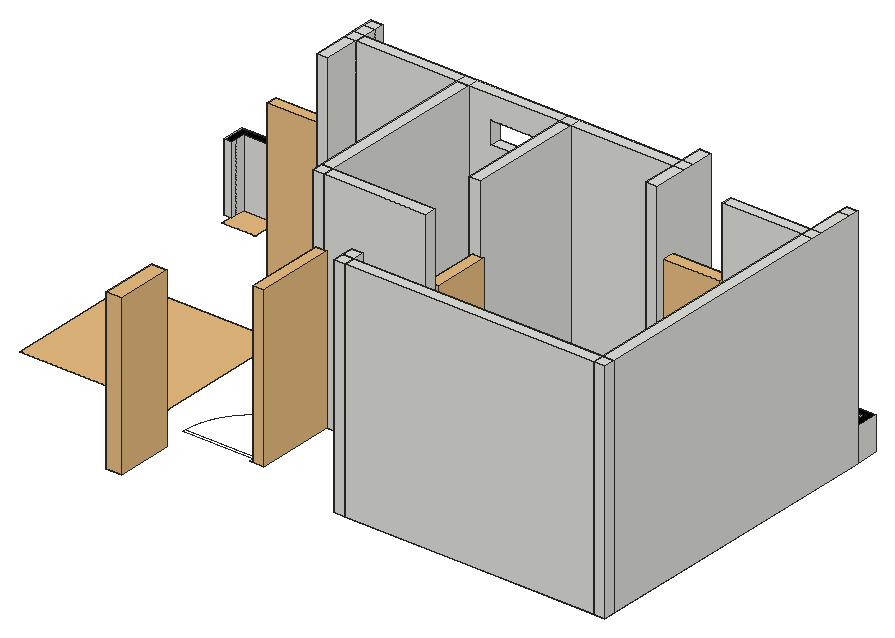
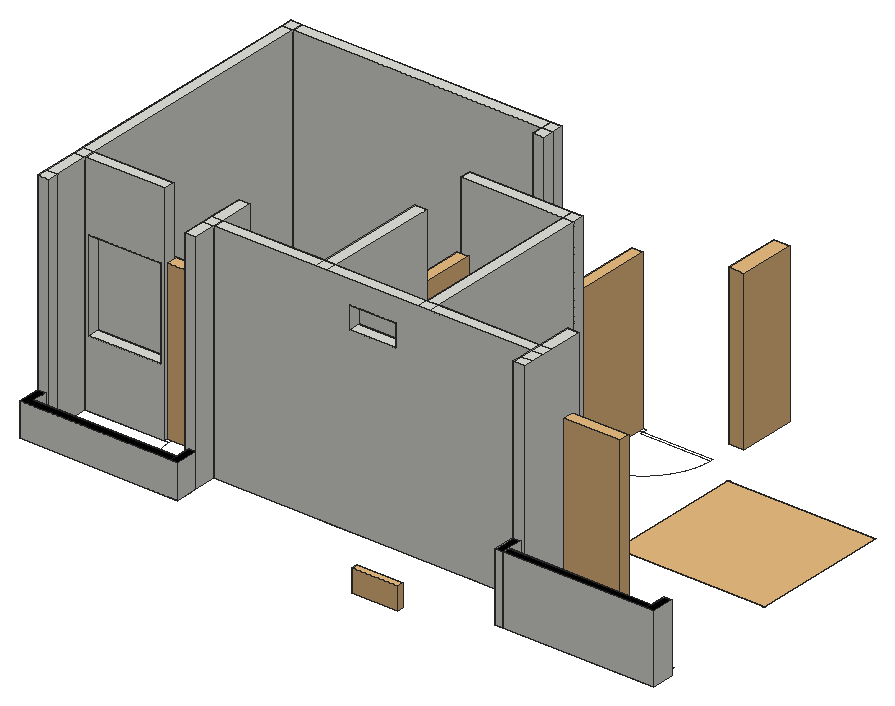
# SketchUp Ruby script. Lengths in inches.
U = 1.inch
M = Sketchup.active_model
def pt(a) = Geom::Point3d.new(a.map { |v| v * U })
def face(e, loops, mat)
  f = e.add_face(loops[0].map { |a| pt(a) })
  loops[1..].each { |l| e.add_face(l.map { |a| pt(a) }).erase! }
  f.material = f.back_material = mat if mat
  f
end
# faces: each face lists its corners as indices into pts; further lists are holes
def faces(e, pts, list, mat = nil) = list.each { |f| face(e, (f[0].is_a?(Array) ? f : [f]).map { |l| l.map { |i| pts[i] } }, mat) }
# xy, xz, yz: faces in a plane at the given z, y or x. An outline is a flat list of corners, or four numbers for a rectangle; further outlines are holes
def ring(l) = l.size == 4 ? [[l[0], l[1]], [l[2], l[1]], [l[2], l[3]], [l[0], l[3]]] : l.each_slice(2).to_a
def flat(e, list, mat, &to3) = list.each { |f| face(e, (f[0].is_a?(Array) ? f : [f]).map { |l| ring(l).map { |u, v| to3.(u, v) } }, mat) }
def xy(e, z, list, mat = nil) = flat(e, list, mat) { |x, y| [x, y, z] }
def xz(e, y, list, mat = nil) = flat(e, list, mat) { |x, z| [x, y, z] }
def yz(e, x, list, mat = nil) = flat(e, list, mat) { |y, z| [x, y, z] }
def lines(e, pts, list) = list.each { |a, b| e.add_line(pt(pts[a]), pt(pts[b])) }
# prism: a flat outline (further loops are holes) pulled along v
def prism(e, loops, v, mat = nil)
  f = face(e, loops, mat); d = Geom::Vector3d.new(v.map { |x| x * U })
  f.pushpull(f.normal.samedirection?(d) ? d.length : -d.length)
end
def box(e, o, s, mat = nil) = prism(e, [[o, [o[0] + s[0], o[1], o[2]], [o[0] + s[0], o[1] + s[1], o[2]], [o[0], o[1] + s[1], o[2]]]], [0, 0, s[2]], mat)
def at(x, y, z, deg = 0) = Geom::Transformation.translation(pt([x, y, z])) * Geom::Transformation.rotation(ORIGIN, Z_AXIS, deg.degrees)
def axes(o, x, y, z) = Geom::Transformation.new([*x, 0, *y, 0, *z, 0, *pt(o).to_a, 1])
def part(name) = M.definitions.add(name)
# library, detail: a bought-in or finely detailed component or shape, given as its bounding box
def library(name, o, s) = part(name).tap { |d| box(d.entities, o, s) }
def detail(e, o, s) = box(e.add_group.entities, o, s)
def put(e, d, t, mat = nil) = e.add_instance(d, t).tap { |i| i.material = mat if mat }
def group(e, t, mat = nil) = e.add_group.tap { |g| g.transformation = t; g.material = mat if mat }.entities
root = M.entities
M.materials.add("M09_Shadow_Night").color = [0, 0, 0]
c1 = library("Group\#49",[0,0,0],[8.31,30,84])
c2 = part("EGWF")
p = [[2.59,-3.49,0],[2.59,-3.09,0],[2.85,-3.09,0],[2.85,-2.99,0],[3.58,-2.99,0],[3.58,-3.49,0],
  [2.59,3.49,0],[2.59,3.09,0],[2.85,3.09,0],[2.85,2.99,0],[3.58,2.99,0],[3.58,3.49,0],
  [-3.58,-3.09,0],[2.59,-2.82,0],[-3.58,-2.82,0],[2.2,3.07,0],[1.81,3.04,0],[1.42,2.97,0],
  [1.03,2.89,0],[0.66,2.78,0],[0.29,2.64,0],[-0.07,2.48,0],[-0.42,2.3,0],[-0.76,2.1,0],
  [-1.08,1.875,0],[-1.39,1.63,0],[-1.68,1.37,0],[-1.96,1.09,0],[-2.21,0.79,0],[-2.45,0.48,0],
  [-2.67,0.15,0],[-2.86,-0.1875,0],[-3.04,-0.54,0],[-3.1875,-0.9,0],[-3.32,-1.28,0],[-3.42,-1.66,0],
  [-3.5,-2.04,0],[-3.55,-2.43,0]]
lines(c2.entities,p,[[0,1],[1,2],[2,3],[3,4],[4,5],[5,0],[6,7],[7,8],[8,9],[9,10],[10,11],[11,6],
  [1,12],[13,14],[1,13],[12,14],[7,15],[15,16],[16,17],[17,18],[18,19],[19,20],[20,21],[21,22],
  [22,23],[23,24],[24,25],[25,26],[26,27],[27,28],[28,29],[29,30],[30,31],[31,32],[32,33],[33,34],
  [34,35],[35,36],[36,37],[37,14]])
c3 = library("Group\#51",[0,0,0],[6.9375,42,86.5])
c4 = library("double bed",[-999.9375,-1062.5,0],[1999.875,2125,0.01])
c5 = library("JEEW",[-211.14,-299.86,0],[422.28,599.72,0.01])
c6 = part("tgr")
p = [[-2.37,-3.35,0],[-2.37,-2.82,0],[-2.73,-2.82,0],[-2.73,-2.68,0],[-3.71,-2.68,0],[-3.71,-3.35,0],
  [-2.37,3.35,0],[-2.37,2.82,0],[-2.73,2.82,0],[-2.73,2.68,0],[-3.71,2.68,0],[-3.71,3.35,0],
  [3.71,-2.82,0],[-2.37,-2.46,0],[3.71,-2.46,0],[3.7,-2.46,0],[3.63,-2.07,0],[3.53,-1.68,0],
  [3.41,-1.3,0],[3.27,-0.93,0],[3.1,-0.57,0],[2.91,-0.22,0],[2.7,0.12,0],[2.46,0.4375,0],
  [2.21,0.74,0],[1.93,1.03,0],[1.64,1.3,0],[1.33,1.55,0],[1.01,1.79,0],[0.67,1.99,0],
  [0.32,2.18,0],[-0.04,2.35,0],[-0.41,2.49,0],[-0.8,2.6,0],[-1.18,2.69,0],[-1.58,2.76,0],
  [-1.97,2.8,0]]
lines(c6.entities,p,[[0,1],[1,2],[2,3],[3,4],[4,5],[5,0],[6,7],[7,8],[8,9],[9,10],[10,11],[11,6],
  [1,12],[13,14],[1,13],[12,14],[15,16],[16,17],[17,18],[18,19],[19,20],[20,21],[21,22],[22,23],
  [23,24],[24,25],[25,26],[26,27],[27,28],[28,29],[29,30],[30,31],[31,32],[32,33],[33,34],[34,35],
  [35,36],[36,7]])
c7 = library("lcd-01",[-577.99,-134.75,0],[1155.98,269.5,0.01])
c8 = part("Group\#126")
xy(c8.entities,0,[[-138,-162.42,-132,-156.42],[-132,-162.42,0,-156.42],[0,-162.42,6,-156.42],[-138,-156.42,-132,-150.42],[0,-156.42,6,-24.42],
  [-42,-24.42,0,-18.42],[0,-24.42,6,-18.42],[0,-18.42,6,0],[0,0,6,5.51]])
xy(c8.entities,36,[[-40,-24.42,-2,-18.42]])
xy(c8.entities,84,[[-40,-24.42,-2,-18.42]])
xy(c8.entities,120,[[-138,-162.42,-132,-156.42],[-132,-162.42,0,-156.42],[0,-162.42,6,-156.42],[-138,-156.42,-132,-150.42],[0,-156.42,6,-24.42],
  [-42,-24.42,0,-18.42],[0,-24.42,6,-18.42],[0,-18.42,6,0],[0,0,6,5.51]])
xz(c8.entities,-162.42,[[-138,0,-132,120],[-132,0,0,120],[0,0,6,120]])
xz(c8.entities,-156.42,[[-138,0,-132,120],[-132,0,0,120],[0,0,6,120]])
xz(c8.entities,-150.42,[[-138,0,-132,120]])
xz(c8.entities,-24.42,[[[-42,0,0,120],[-40,36,-2,84]]])
xz(c8.entities,-18.42,[[[-42,0,0,120],[-40,36,-2,84]]])
xz(c8.entities,5.51,[[0,0,6,120]])
yz(c8.entities,-138,[[-162.42,0,-156.42,120],[-156.42,0,-150.42,120]])
yz(c8.entities,-132,[[-162.42,0,-156.42,120],[-156.42,0,-150.42,120]])
yz(c8.entities,-42,[[-24.42,0,-18.42,120]])
yz(c8.entities,-40,[[-24.42,36,-18.42,84]])
yz(c8.entities,-2,[[-24.42,36,-18.42,84]])
yz(c8.entities,0,[[-162.42,0,-156.42,120],[-156.42,0,-24.42,120],[-24.42,0,-18.42,120],[-18.42,0,0,120],[0,0,5.51,120]])
yz(c8.entities,6,[[-162.42,0,-156.42,120],[-156.42,0,5.51,120]])
c9 = part("G5GTGTGT")
p = [[0.52,4.97,0],[0.52,-4.97,0],[0.36,-4.97,0],[0.36,4.97,0],[-0.08,-4.53,0],[-0.08,4.53,0],
  [0.33,4.97,0],[0.3,4.97,0],[0.28,4.96,0],[0.25,4.96,0],[0.22,4.95,0],[0.2,4.94,0],
  [0.17,4.93,0],[0.15,4.92,0],[0.12,4.9,0],[0.1,4.89,0],[0.08,4.87,0],[0.06,4.85,0],
  [0.04,4.83,0],[0.02,4.8125,0],[0,4.79,0],[-0.01,4.77,0],[-0.03,4.74,0],[-0.04,4.72,0],
  [-0.05,4.69,0],[-0.0625,4.67,0],[-0.07,4.64,0],[-0.08,4.61,0],[-0.08,4.59,0],[-0.08,4.56,0],
  [-0.08,-4.56,0],[-0.08,-4.59,0],[-0.08,-4.61,0],[-0.07,-4.64,0],[-0.0625,-4.67,0],[-0.05,-4.69,0],
  [-0.04,-4.72,0],[-0.03,-4.74,0],[-0.01,-4.77,0],[0,-4.79,0],[0.02,-4.8125,0],[0.04,-4.83,0],
  [0.06,-4.85,0],[0.08,-4.87,0],[0.1,-4.89,0],[0.12,-4.9,0],[0.15,-4.92,0],[0.17,-4.93,0],
  [0.2,-4.94,0],[0.22,-4.95,0],[0.25,-4.96,0],[0.28,-4.96,0],[0.3,-4.97,0],[0.33,-4.97,0],
  [-0.08,-1.38,0],[-0.52,-1.38,0],[-0.08,1.38,0],[-0.52,1.38,0]]
lines(c9.entities,p,[[0,1],[1,2],[2,3],[3,0],[4,5],[3,6],[6,7],[7,8],[8,9],[9,10],[10,11],[11,12],
  [12,13],[13,14],[14,15],[15,16],[16,17],[17,18],[18,19],[19,20],[20,21],[21,22],[22,23],[23,24],
  [24,25],[25,26],[26,27],[27,28],[28,29],[29,5],[4,30],[30,31],[31,32],[32,33],[33,34],[34,35],
  [35,36],[36,37],[37,38],[38,39],[39,40],[40,41],[41,42],[42,43],[43,44],[44,45],[45,46],[46,47],
  [47,48],[48,49],[49,50],[50,51],[51,52],[52,53],[53,2],[54,55],[56,57],[55,57]])
c10 = part("Group\#15")
xy(c10.entities,0,[[60,-108.67,66,-102.67],[66,-108.67,120.4,-102.67],[60,-102.67,66,-12.67],[114.4,-72.67,120.4,-12.67],[0,-30.67,6,-12.67],
  [174.4,-30.67,180.4,-12.67],[0,-12.67,6,-6.67],[6,-12.67,60,-6.67],[60,-12.67,66,-6.67],[66,-12.67,114.4,-6.67],
  [114.4,-12.67,120.4,-6.67],[120.4,-12.67,174.4,-6.67],[174.4,-12.67,180.4,-6.67],[0,-6.67,6,0],[174.4,-6.67,180.4,5.26],
  [0,0,6,5.26]])
xy(c10.entities,96,[[78,-12.67,102.4,-6.67]])
xy(c10.entities,108,[[78,-12.67,102.4,-6.67]])
xy(c10.entities,120,[[60,-108.67,66,-102.67],[66,-108.67,120.4,-102.67],[60,-102.67,66,-12.67],[114.4,-72.67,120.4,-12.67],[0,-30.67,6,-12.67],
  [174.4,-30.67,180.4,-12.67],[0,-12.67,6,-6.67],[6,-12.67,60,-6.67],[60,-12.67,66,-6.67],[66,-12.67,114.4,-6.67],
  [114.4,-12.67,120.4,-6.67],[120.4,-12.67,174.4,-6.67],[174.4,-12.67,180.4,-6.67],[0,-6.67,6,0],[174.4,-6.67,180.4,5.26],
  [0,0,6,5.26]])
xz(c10.entities,-108.67,[[60,0,66,120],[66,0,120.4,120]])
xz(c10.entities,-102.67,[[60,0,66,120],[66,0,120.4,120]])
xz(c10.entities,-72.67,[[114.4,0,120.4,120]])
xz(c10.entities,-30.67,[[0,0,6,120],[174.4,0,180.4,120]])
xz(c10.entities,-12.67,[[6,0,60,120],[60,0,66,120],[[66,0,114.4,120],[78,96,102.4,108]],[114.4,0,120.4,120],[120.4,0,174.4,120]])
xz(c10.entities,-6.67,[[[6,0,174.4,120],[78,96,102.4,108]]])
xz(c10.entities,5.26,[[0,0,6,120],[174.4,0,180.4,120]])
yz(c10.entities,0,[[-30.67,0,5.26,120]])
yz(c10.entities,6,[[-30.67,0,-12.67,120],[-12.67,0,-6.67,120],[-6.67,0,0,120],[0,0,5.26,120]])
yz(c10.entities,60,[[-108.67,0,-102.67,120],[-102.67,0,-12.67,120]])
yz(c10.entities,66,[[-108.67,0,-102.67,120],[-102.67,0,-12.67,120]])
yz(c10.entities,78,[[-12.67,96,-6.67,108]])
yz(c10.entities,102.4,[[-12.67,96,-6.67,108]])
yz(c10.entities,114.4,[[-72.67,0,-12.67,120]])
yz(c10.entities,120.4,[[-108.67,0,-102.67,120],[-72.67,0,-12.67,120]])
yz(c10.entities,174.4,[[-30.67,0,-12.67,120],[-12.67,0,-6.67,120],[-6.67,0,5.26,120]])
yz(c10.entities,180.4,[[-30.67,0,5.26,120]])
c11 = library("ghgjg",[-265.23,-341.01,0],[530.46,682.02,0.01])
c12 = library("Group\#48",[0,0,0],[6.9375,42,86.5])
c13 = library("Component\#3",[961.32,686.58,0],[54,18,0.01])
c14 = library("Component\#4",[1075.72,686.58,0],[54,18,0.01])
c15 = library("Group\#46",[0,-0.05,0],[30,2.55,24])
c16 = library("TREE-26",[-60.96,-72.91,0],[121.92,134.74,0.01])
c17 = part("Group\#13")
xy(c17.entities,0,[[0,0,4,3.01],[80,0,84,8],[0,3.01,4,8],[0,8,4,12],[4,8,80,12],
  [80,8,84,12]])
xy(c17.entities,36,[[0,0,4,12],[80,0,84,12],[4,8,80,12]],"M09_Shadow_Night")
xz(c17.entities,0,[[0,0,4,36],[80,0,84,36]])
xz(c17.entities,8,[[4,0,80,36]])
xz(c17.entities,12,[[0,0,80,36],[80,0,84,36]])
yz(c17.entities,0,[[0,0,12,36]])
yz(c17.entities,4,[[0,0,3.01,36],[3.01,0,8,36]])
yz(c17.entities,80,[[0,0,8,36],[8,0,12,36]])
yz(c17.entities,84,[[0,0,12,36]])
c18 = part("Group\#16")
xy(c18.entities,0,[[0,0,4,3.74],[80,0,84,8],[0,3.74,4,8],[0,8,4,12],[4,8,80,12],
  [80,8,84,12]])
xy(c18.entities,18,[[0,0,4,12],[80,0,84,0,84,12,4,12,4,8,80,8]],"M09_Shadow_Night")
xz(c18.entities,0,[[0,0,4,18],[80,0,84,18]])
xz(c18.entities,8,[[4,0,80,18]])
xz(c18.entities,12,[[0,0,84,18]])
yz(c18.entities,0,[[0,0,12,18]])
yz(c18.entities,4,[[0,0,3.74,18],[3.74,0,8,18]])
yz(c18.entities,80,[[0,0,8,18]])
yz(c18.entities,84,[[0,0,12,18]])
box(root,[224.2,703.34,246],[54,18,1])
xy(root,246,[[218.2,571.34,362.2,571.34,362.2,739.27,356.2,739.27,356.2,715.34,314.2,715.34,314.2,709.34,356.2,709.34,356.2,577.34,224.2,577.34,224.2,583.34,218.2,583.34]])
put(root,c1,at(121.52,541.34,246))
put(root,c2,axes([239.8,604.34,246],[-6.02515,0,0],[0,6.02515,0],[0,0,6.02515]))
put(root,c2,axes([148.2,604.34,246],[6.02515,0,0],[0,6.02515,0],[0,0,6.02515]))
put(root,c1,axes([222.48,625.34,246],[-1,0,0],[0,-1.4,0],[0,0,1]))
put(root,c3,axes([171.46,625.34,246],[-0.85622,0,0],[0,-1,0],[0,0,0.9711]))
put(root,c4,axes([71.06,633.07,246],[0,-0.03695,0],[-0.03695,0,0],[0,0,0.03695]))
put(root,c4,axes([316.9375,633.07,246],[0,-0.03695,0],[0.03695,0,0],[0,0,0.03695]))
put(root,c5,axes([178.84,644.18,246],[-0.04284,0,0],[0,0.04284,0],[0,0,0.04284]))
put(root,c6,axes([207.6,646.34,246],[-4.47464,0,0],[0,4.47464,0],[0,0,4.47464]))
put(root,c3,axes([225.86,661.34,246],[-0.85622,0,0],[0,-0.71429,0],[0,0,0.9711]))
put(root,c7,axes([158.41,652,246],[0,-0.04,0],[0.04,0,0],[0,0,0.04]))
put(root,c8,at(356.2,733.76,246))
put(root,c9,axes([226.1,681.76,246],[3.62,0,0],[0,3.62,0],[0,0,3.62]))
put(root,c10,at(103.8,734.01,246))
put(root,c11,axes([193.9,707.6,246],[-0.04,0,0],[0,0.04,0],[0,0,0.04]))
put(root,c3,axes([103.8,707.68,246],[0,0.85622,0],[-0.71429,0,0],[0,0,0.97071]))
put(root,c12,axes([314.2,707.68,246],[0,0.85622,0],[-0.71429,0,0],[0,0,0.97071]))
put(root,c13,at(-851.52,16.76,246))
put(root,c14,at(-851.52,16.76,246))
put(root,c15,axes([206.2,725.55,216],[-0.81341,0,0],[0,-1.27878,0],[0,0,0.5]))
put(root,c6,axes([88.8,725.9375,246],[0,4.47464,0],[-4.47464,0,0],[0,0,4.47464]))
put(root,c6,axes([299.2,725.9375,246],[0,4.47464,0],[4.47464,0,0],[0,0,4.47464]))
put(root,c16,axes([38.7,741.86,246],[0,0.1317,0],[0.1317,0,0],[0,0,0.1317]))
put(root,c16,axes([349.66,741.86,246],[0,0.1317,0],[0.1317,0,0],[0,0,0.1317]))
put(root,c17,at(25.8,739.27,246))
put(root,c18,at(278.2,739.27,246))
